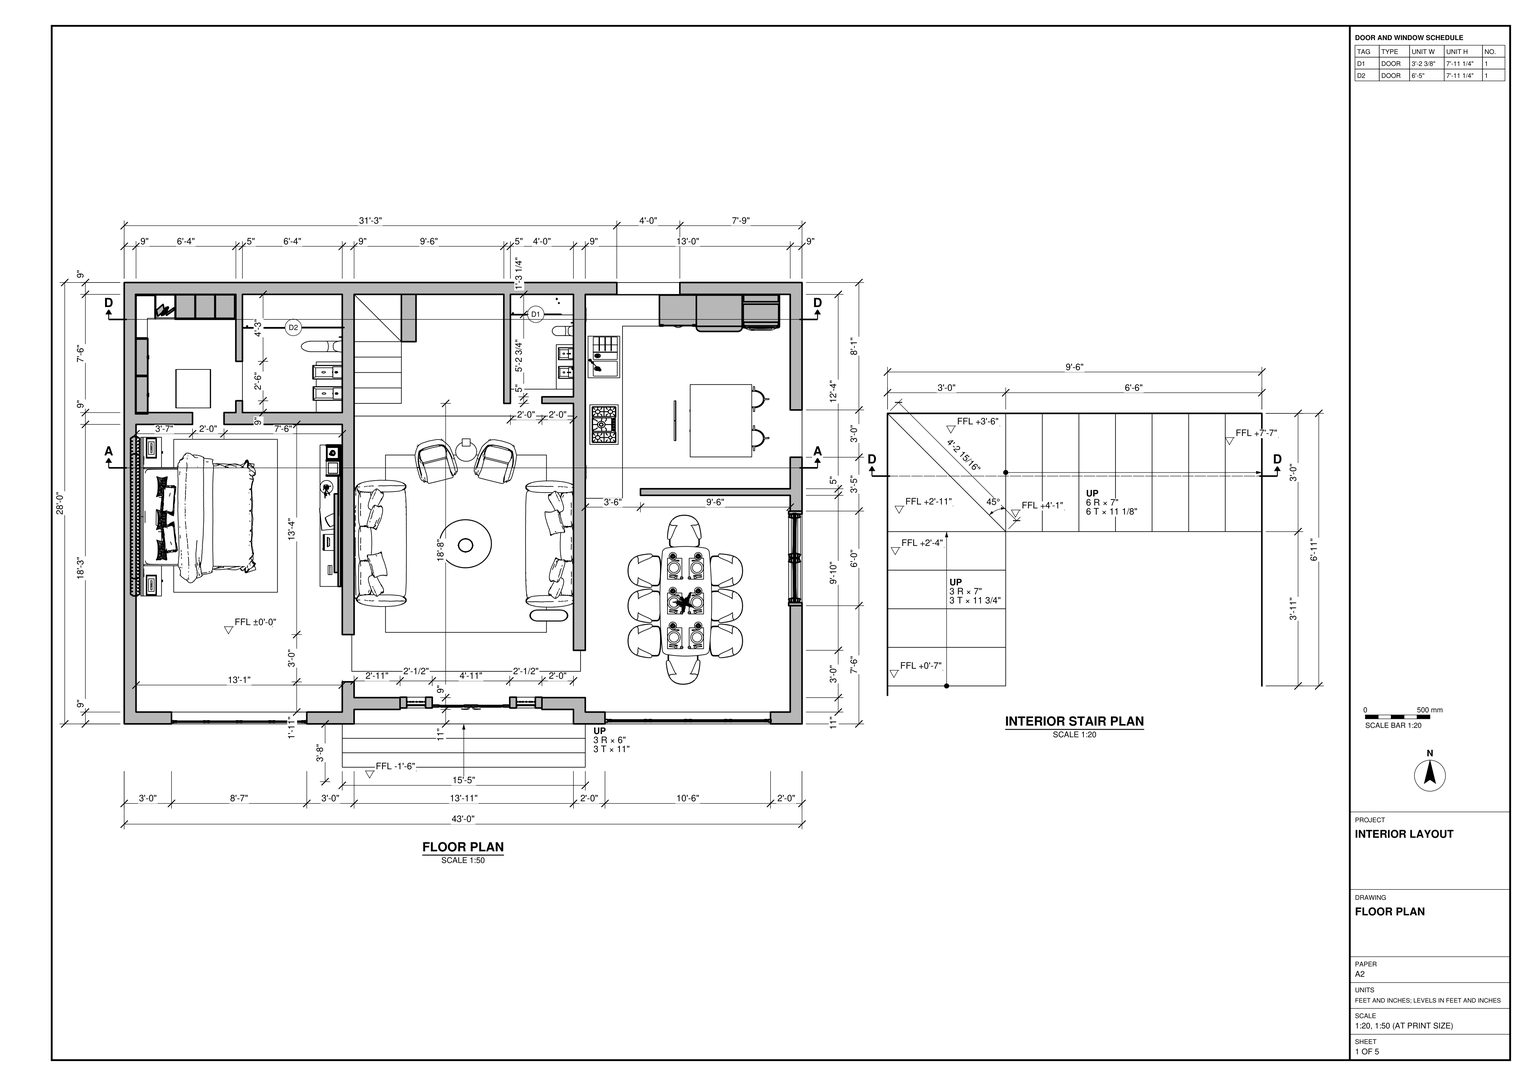
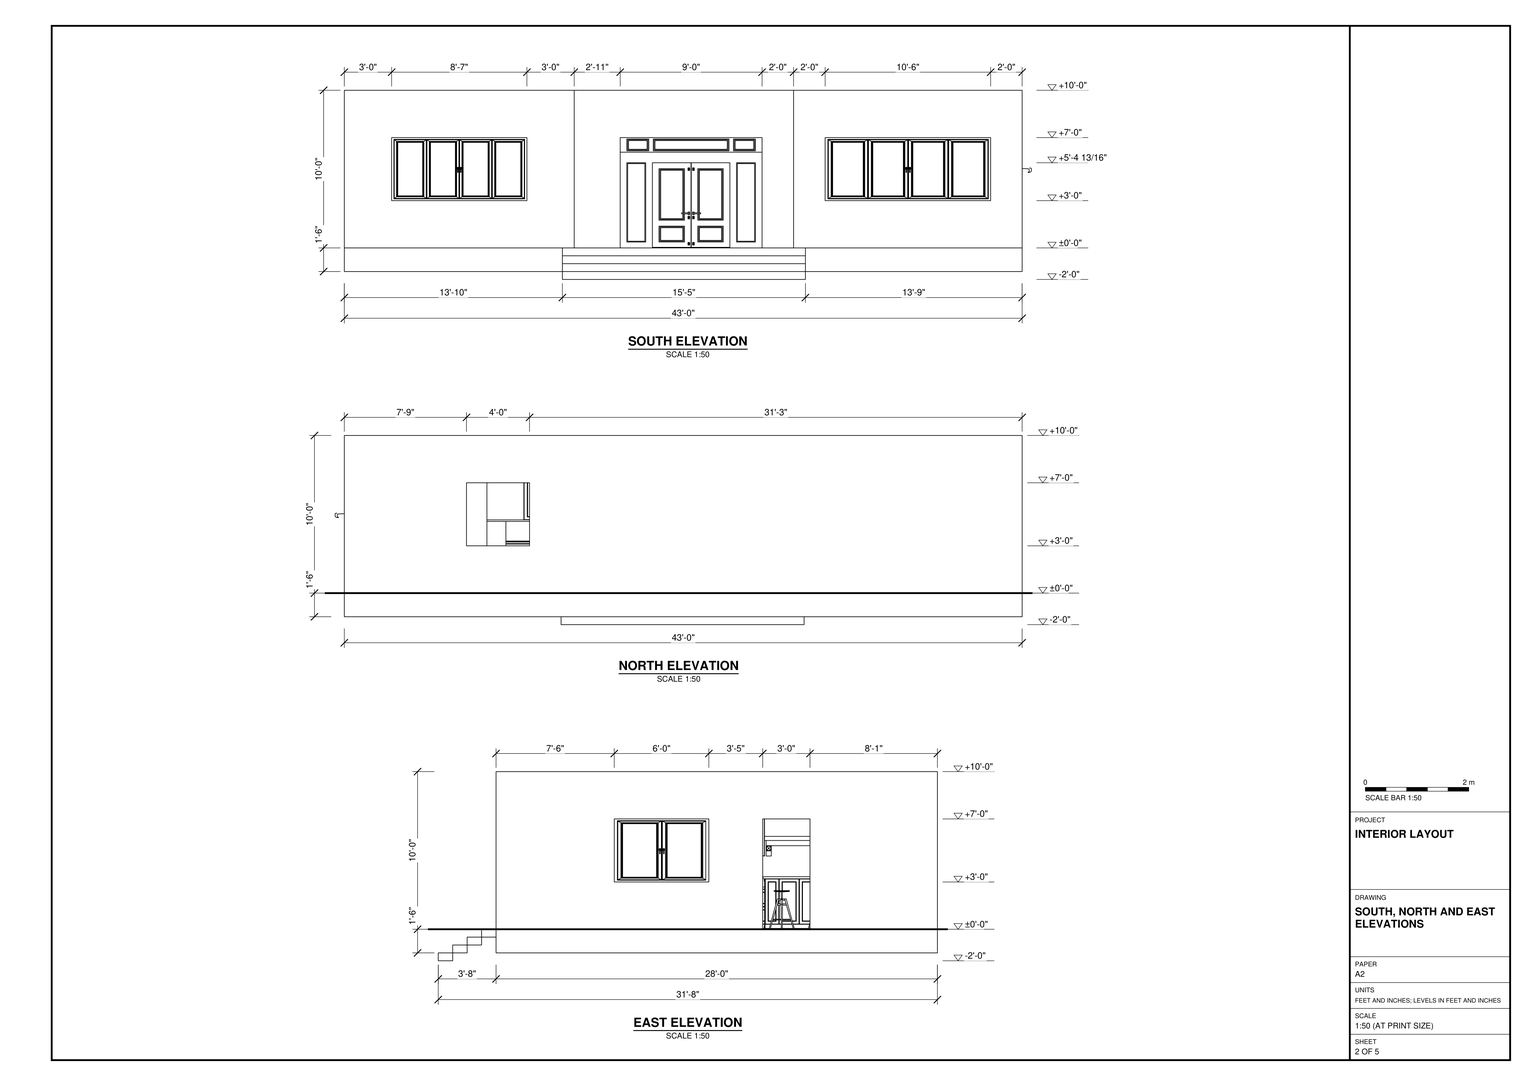
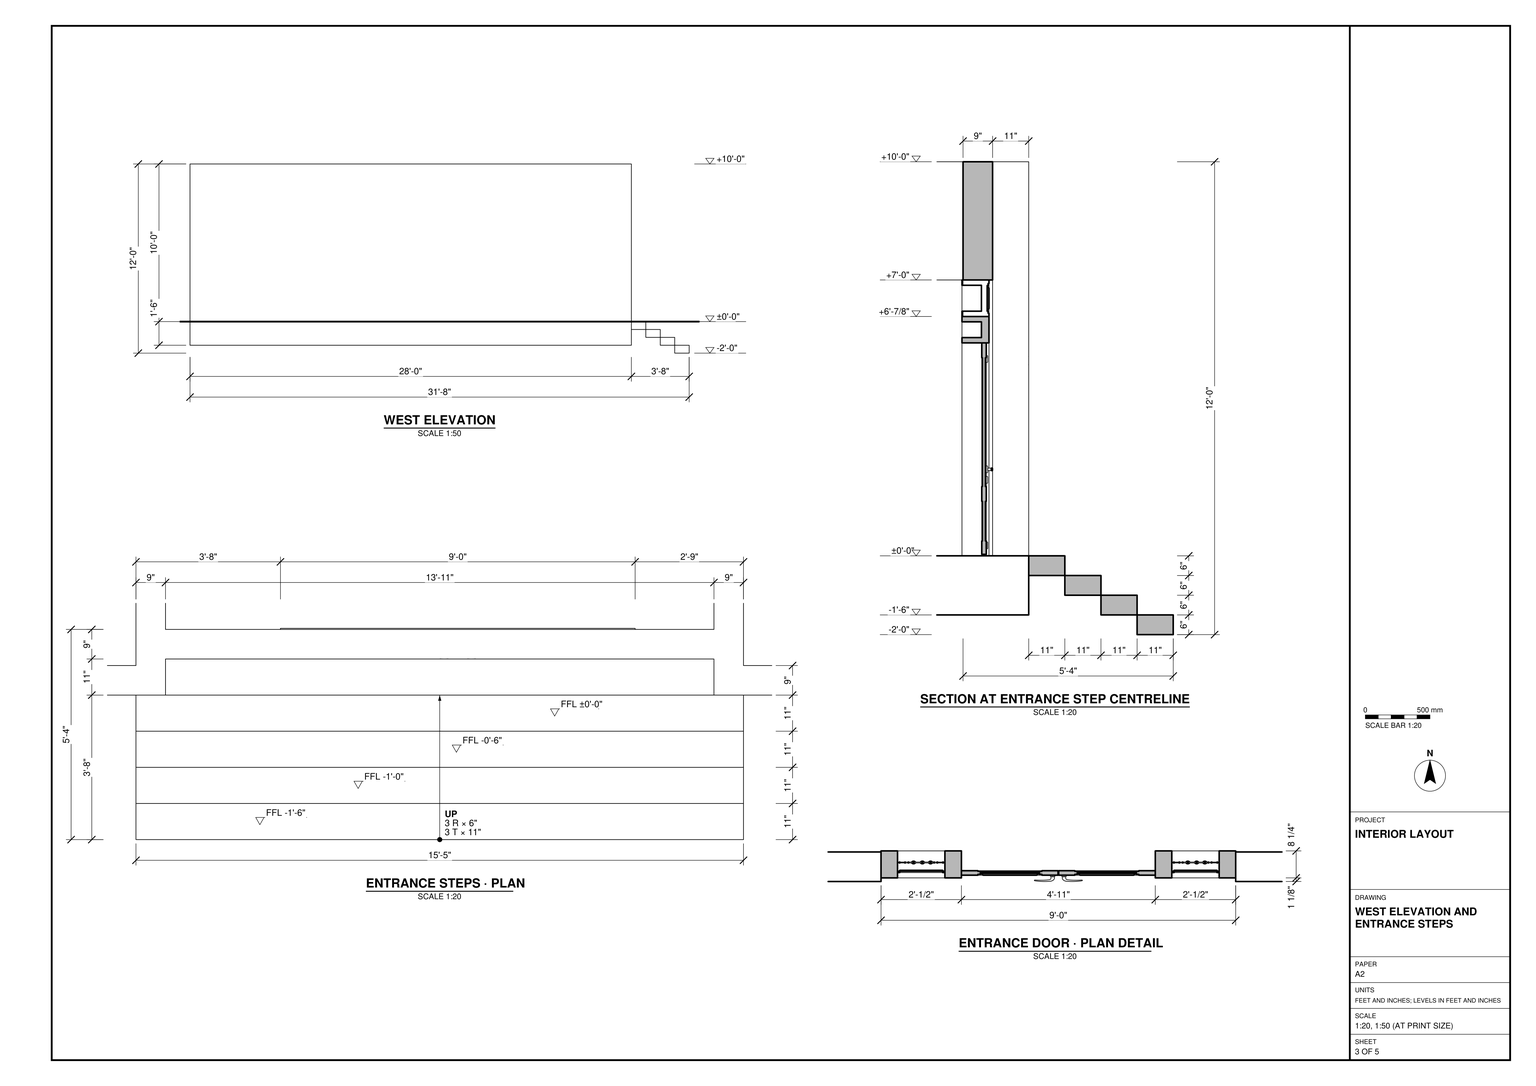
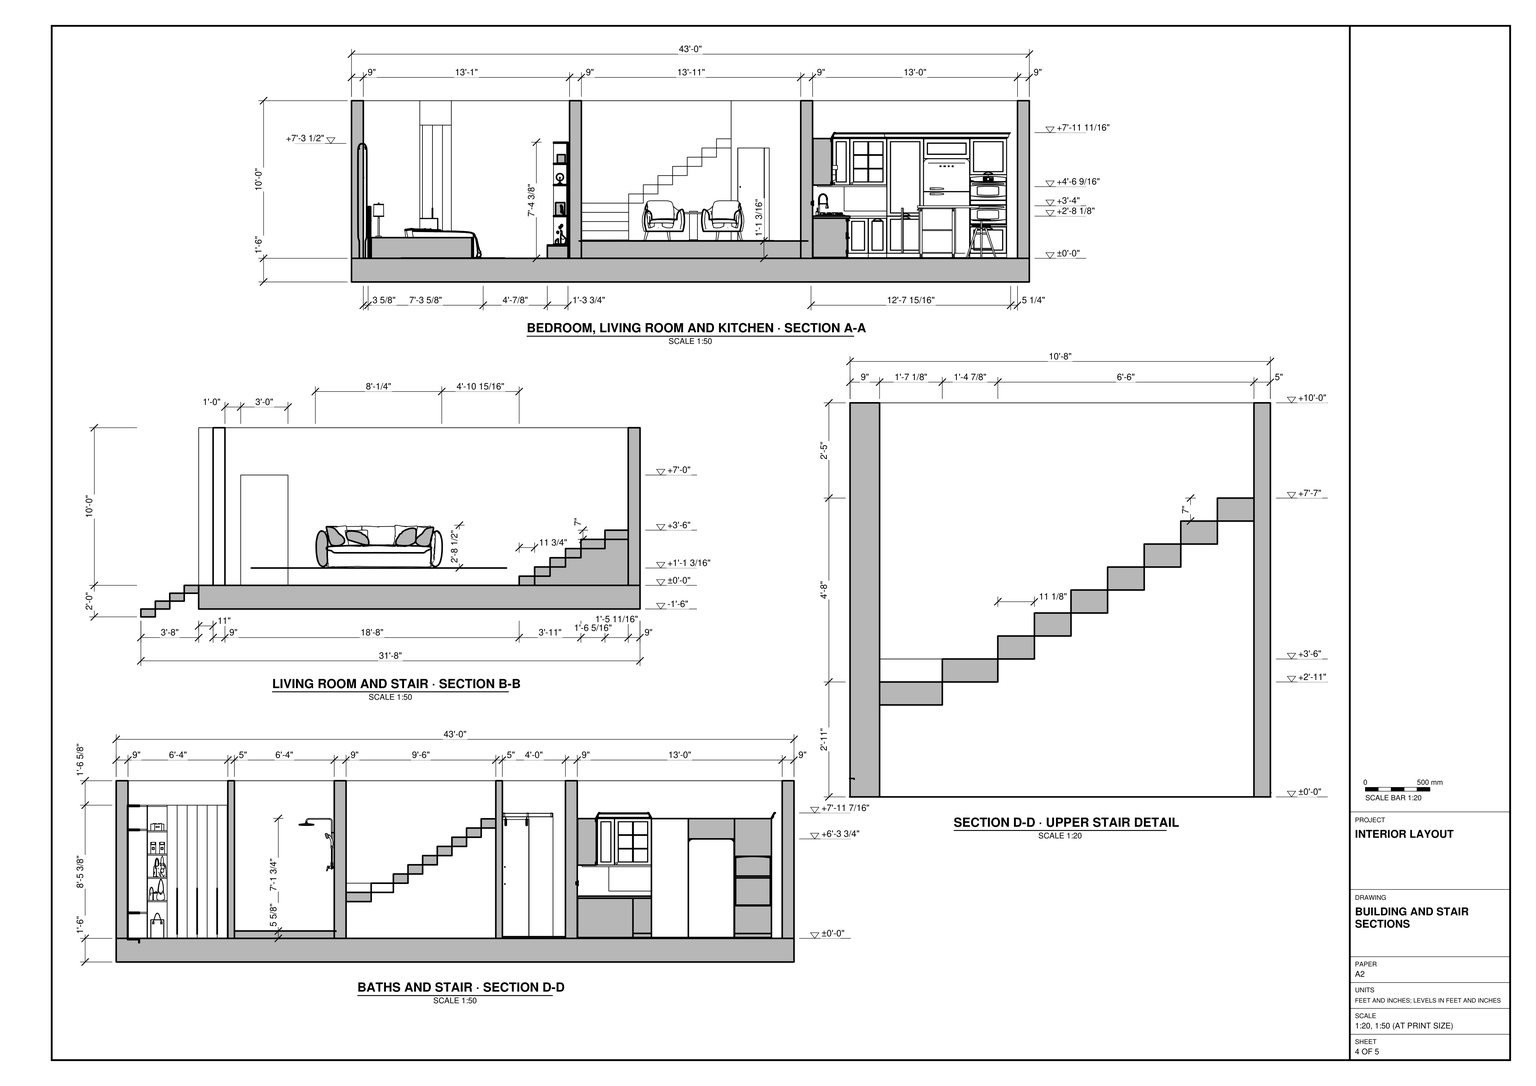
Build the residential interior in SketchUp from task_files/diagram_01.pdf. Work in feet and inches. The complete model measures 43'-7 7/16" along X, 40'-11 11/16" along Y and 12'-0" vertically. Set the finished ground floor at ±0'-0". Distinguish the complete model extents from the 43'-0" by 28'-0" exterior wall footprint on the floor plan.

Model the raised floor slab, the 9" exterior walls and the interior walls at their drawn thicknesses, including the 5" partitions. Form the recessed south entrance with broad steps, paired door leaves, sidelights and a transom. Use the elevations to locate the window units and the openings on the east and north walls. Model the interior stair behind the living area, including the angled treads where the flight turns.

Place the bed with its head against the west wall, bedside units on either side and storage opposite. Fit out the small rooms along the north wall with the storage and sanitary fixtures shown. Arrange the central sofas facing each other across the round table, with the armchairs toward the stair. In the east bay, model the kitchen counters, sink, cooktop, island and stools behind the dining area. Match the footprints and orientations of the dining table, chairs and other main furniture to the plan. Decor and loose items may be any suitable library components.

Keep the shell elements, stairs and each furniture or joinery piece in separate groups or components, and use components for repeated parts. Save one SketchUp model as output_files/furnished_interior_with_entrance_steps_and_turning_stair.skp.

# SketchUp Ruby script. Lengths in inches.
U = 1.inch
M = Sketchup.active_model
def pt(a) = Geom::Point3d.new(a.map { |v| v * U })
def face(e, loops, mat)
  f = e.add_face(loops[0].map { |a| pt(a) })
  loops[1..].each { |l| e.add_face(l.map { |a| pt(a) }).erase! }
  f.material = f.back_material = mat if mat
  f
end
# faces: each face lists its corners as indices into pts; further lists are holes
def faces(e, pts, list, mat = nil) = list.each { |f| face(e, (f[0].is_a?(Array) ? f : [f]).map { |l| l.map { |i| pts[i] } }, mat) }
# xy, xz, yz: faces in a plane at the given z, y or x. An outline is a flat list of corners, or four numbers for a rectangle; further outlines are holes
def ring(l) = l.size == 4 ? [[l[0], l[1]], [l[2], l[1]], [l[2], l[3]], [l[0], l[3]]] : l.each_slice(2).to_a
def flat(e, list, mat, &to3) = list.each { |f| face(e, (f[0].is_a?(Array) ? f : [f]).map { |l| ring(l).map { |u, v| to3.(u, v) } }, mat) }
def xy(e, z, list, mat = nil) = flat(e, list, mat) { |x, y| [x, y, z] }
def xz(e, y, list, mat = nil) = flat(e, list, mat) { |x, z| [x, y, z] }
def yz(e, x, list, mat = nil) = flat(e, list, mat) { |y, z| [x, y, z] }
def lines(e, pts, list) = list.each { |a, b| e.add_line(pt(pts[a]), pt(pts[b])) }
# prism: a flat outline (further loops are holes) pulled along v
def prism(e, loops, v, mat = nil)
  f = face(e, loops, mat); d = Geom::Vector3d.new(v.map { |x| x * U })
  f.pushpull(f.normal.samedirection?(d) ? d.length : -d.length)
end
def box(e, o, s, mat = nil) = prism(e, [[o, [o[0] + s[0], o[1], o[2]], [o[0] + s[0], o[1] + s[1], o[2]], [o[0], o[1] + s[1], o[2]]]], [0, 0, s[2]], mat)
def at(x, y, z, deg = 0) = Geom::Transformation.translation(pt([x, y, z])) * Geom::Transformation.rotation(ORIGIN, Z_AXIS, deg.degrees)
def axes(o, x, y, z) = Geom::Transformation.new([*x, 0, *y, 0, *z, 0, *pt(o).to_a, 1])
def part(name) = M.definitions.add(name)
# library, detail: a bought-in or finely detailed component or shape, given as its bounding box
def library(name, o, s) = part(name).tap { |d| box(d.entities, o, s) }
def detail(e, o, s) = box(e.add_group.entities, o, s)
def put(e, d, t, mat = nil) = e.add_instance(d, t).tap { |i| i.material = mat if mat }
def group(e, t, mat = nil) = e.add_group.tap { |g| g.transformation = t; g.material = mat if mat }.entities
root = M.entities
M.materials.add("02").color = [126, 126, 126]
M.materials.add("9225458-white-marble-texture-background-High-resolution-scan").color = [224, 224, 224]
M.materials.add("Hairline Grey").color = [62, 62, 62]
M.materials.add("Lisanne_Boots").color = [231, 232, 226]
M.materials.add("WD-03").color = [28, 27, 25]
M.materials.add("WoodPlanksClean0025_9_S").color = [124, 95, 68]
M.materials.add("[0100_SteelBlue]").color = [246, 244, 236]
M.materials.add("[0131_Silver]").color = [192, 192, 192]
M.materials.add("[Aluminum]").color = [179, 179, 179]
M.materials.add("[Blacktop Old 01]").color = [132, 136, 139]
M.materials.add("[Carrera Marble]").color = [207, 207, 207]
M.materials.add("[Granite Brown]").color = [126, 104, 91]
M.materials.add("[Roofing Slate Tan]").color = [200, 175, 128]
M.materials.add("[Slate Light Tile]").color = [54, 54, 54]
M.materials.add("[Stone Vein Gray]").color = [166, 165, 165]
M.materials.add("[Tile Large Brown]").color = [195, 178, 159]
M.materials.add("[Translucent Glass Gray]").color = [128, 128, 128]
M.materials["[Translucent Glass Gray]"].alpha = 0.5
M.materials.add("trees-164929_960_1").color = [98, 98, 98]
c1 = library("K-3091 Purist(R) Mirrored Cabinet",[0,-6.88,-2.03],[25.45,6.88,38.03])
c2 = library("Sink",[-425.26,-17.96,-2.45],[19.83,19.83,15.37])
c3 = library("CS761DT5",[0,0,0],[27.72,16.22,33.63])
c4 = library("SHOWER",[23.01,60.26,14.57],[13.03,23.97,40.35])
c5 = part("Bar")
prism(c5.entities,[[[0,0.25,0.5],[0,0.47,0.375],[0,0.47,0.125],[0,0.25,0],[0,0.03,0.125],[0,0.03,0.375]]],[11.5,0,0])
c6 = part("End")
xy(c6.entities,0,[[0,0.25,0.875,1.5]],"[0131_Silver]")
xy(c6.entities,0.5,[[0,0.25,0.875,1.5]],"[0131_Silver]")
xz(c6.entities,0.03,[[0,0.125,0.25,0.375]],"[0131_Silver]")
xz(c6.entities,0.47,[[0.25,0.125,0.875,0.375]],"[0131_Silver]")
xz(c6.entities,1.5,[[0,0,0.875,0.5]],"[0131_Silver]")
yz(c6.entities,0,[[0.25,0,0.03,0.125,0.03,0.375,0.25,0.5,1.5,0.5,1.5,0]],"[0131_Silver]")
yz(c6.entities,0.25,[[0.25,0,0.47,0.125,0.47,0.375,0.25,0.5,0.03,0.375,0.03,0.125]],"[0131_Silver]")
yz(c6.entities,0.875,[[0.25,0,1.5,0,1.5,0.5,0.25,0.5,0.47,0.375,0.47,0.125]],"[0131_Silver]")
p = [[0,0.25,0],[0.25,0.25,0],[0.25,0.03,0.125],[0,0.03,0.125],[0.875,0.25,0],[0.875,0.47,0.125],
  [0.25,0.47,0.125],[0,0.03,0.375],[0.25,0.03,0.375],[0.25,0.25,0.5],[0,0.25,0.5],[0.875,0.47,0.375],
  [0.875,0.25,0.5],[0.25,0.47,0.375]]
faces(c6.entities,p,[[0,1,2,3],[4,5,6,1],[7,8,9,10],[11,12,9,13]],"[0131_Silver]")
c7 = part("Drawer Pull\#2")
put(c7.entities,c5,axes([0.25,0,0],[1.16,0,0],[0,0.76843,0],[0,0,1]),"[0131_Silver]")
put(c7.entities,c6,axes([0,0,0],[1,0,0],[0,1.02284,0],[0,0,1]))
put(c7.entities,c6,axes([13.84,0,0],[-1,0,0],[0,1.02284,0],[0,0,1]))
c8 = part("NUT")
prism(c8.entities,[[[0.34,0,0],[0,0.2,0],[0,0.6,0],[0.34,0.79,0],[0.6875,0.6,0],[0.6875,0.2,0]]],[0,0,0.25])
c9 = part("BOLT HEAD")
yz(c9.entities,0,[[0.34,-0.14,0.27,-0.12,0.22,-0.07,0.21,0,0.22,0.07,0.27,0.12,0.34,0.14,0.41,0.12,0.46,0.07,0.48,0,0.46,-0.07,0.41,-0.12]])
p = [[0.1875,0.05,-0.17],[0,0.22,-0.07],[0,0.27,-0.12],[0.1875,0.17,-0.3],[0,0.34,-0.14],[0.1875,0.34,-0.34],
  [0,0.41,-0.12],[0.1875,0.52,-0.3],[0,0.46,-0.07],[0.1875,0.64,-0.17],[0.1875,0,0],[0,0.21,0],
  [0,0.48,0],[0.1875,0.6875,0],[0.1875,0.05,0.17],[0,0.22,0.07],[0,0.46,0.07],[0.1875,0.64,0.17],
  [0.1875,0.17,0.3],[0,0.27,0.12],[0.1875,0.34,0.34],[0,0.34,0.14],[0.1875,0.52,0.3],[0,0.41,0.12]]
faces(c9.entities,p,[[0,1,2,3],[3,2,4,5],[5,4,6,7],[7,6,8,9],[10,11,1,0],[9,8,12,13],[14,15,11,10],[13,12,16,17],
  [18,19,15,14],[20,21,19,18],[22,23,21,20],[17,16,23,22]])
c10 = part("Group\#42")
xy(c10.entities,0,[[0.33,0.41,0.33,0.75,0,0.97,0,1.4375,0.19,1.4375,0.19,1.07,0.52,0.85,0.52,0.41],[0,1.4375,0,1.91,0.33,2.12,0.33,2.46,0.52,2.46,0.52,2.02,0.19,1.8,0.19,1.4375]],"[Aluminum]")
xy(c10.entities,4.24,[[0.625,0,1.0625,0.85],[0.625,2.02,1.0625,2.875]],"[Aluminum]")
xy(c10.entities,4.43,[[0.6,0,1.0625,0.75],[0.6,2.12,1.0625,2.875]],"[Aluminum]")
xy(c10.entities,4.57,[[0.58,1.07,1.0625,1.4375],[0.58,1.4375,1.0625,1.8]],"[Aluminum]")
xy(c10.entities,4.76,[[0.56,0.97,1.0625,1.4375],[0.56,1.4375,1.0625,1.91]],"[Aluminum]")
xz(c10.entities,0,[[0.33,0.41,0.52,0.41,0.52,4.14,0.53,4.1875,0.57,4.23,0.625,4.24,1.0625,4.24,1.0625,4.43,0.6,4.43,0.47,4.4,0.36,4.29,0.33,4.16]],"[Aluminum]")
xz(c10.entities,2.875,[[0.33,0.41,0.33,4.16,0.36,4.29,0.47,4.4,0.6,4.43,1.0625,4.43,1.0625,4.24,0.625,4.24,0.57,4.23,0.53,4.1875,0.52,4.14,0.52,0.41]],"[Aluminum]")
yz(c10.entities,0,[[0.97,0,1.4375,4.2],[1.4375,0,1.91,4.2]],"[Aluminum]")
yz(c10.entities,0.19,[[1.07,0,1.4375,4.18],[1.4375,0,1.8,4.18]],"[Aluminum]")
yz(c10.entities,0.33,[[0.41,0,0,0.41,0,4.16,0.75,4.16,0.75,0],[2.12,0,2.12,4.16,2.875,4.16,2.875,0.41,2.46,0]],"[Aluminum]")
yz(c10.entities,0.52,[[0.41,0,0.85,0,0.85,4.14,0,4.14,0,0.41],[2.02,0,2.46,0,2.875,0.41,2.875,4.14,2.02,4.14]],"[Aluminum]")
yz(c10.entities,1.0625,[[0,4.24,0.85,4.24,1.07,4.57,1.4375,4.57,1.4375,4.76,0.97,4.76,0.75,4.43,0,4.43],[2.02,4.24,2.875,4.24,2.875,4.43,2.12,4.43,1.91,4.76,1.4375,4.76,1.4375,4.57,1.8,4.57]],"[Aluminum]")
p = [[0.33,0,0.41],[0.33,0.41,0],[0.52,0.41,0],[0.52,0,0.41],[0,0.97,0],[0.33,0.75,0],
  [0.33,0.75,4.16],[0,0.97,4.2],[0.52,0.85,0],[0.19,1.07,0],[0.19,1.07,4.18],[0.52,0.85,4.14],
  [0.19,1.8,0],[0.52,2.02,0],[0.52,2.02,4.14],[0.19,1.8,4.18],[0.33,2.12,0],[0,1.91,0],
  [0,1.91,4.2],[0.33,2.12,4.16],[0.33,2.46,0],[0.33,2.875,0.41],[0.52,2.875,0.41],[0.52,2.46,0],
  [0.52,0,4.14],[0.53,0.85,4.1875],[0.53,0,4.1875],[0.24,1.07,4.36],[0.53,2.02,4.1875],[0.24,1.8,4.36],
  [0.52,2.875,4.14],[0.53,2.875,4.1875],[0.33,0,4.16],[0.36,0,4.29],[0.36,0.75,4.29],[0.57,0.85,4.23],
  [0.57,0,4.23],[0.625,0.85,4.24],[0.625,0,4.24],[0.07,0.97,4.46],[0.4,1.07,4.52],[0.58,1.07,4.57],
  [1.0625,1.07,4.57],[1.0625,0.85,4.24],[0.07,1.4375,4.46],[0,1.4375,4.2],[0.19,1.4375,4.18],[0.24,1.4375,4.36],
  [0.07,1.91,4.46],[0.57,2.02,4.23],[0.4,1.8,4.52],[0.625,2.02,4.24],[0.58,1.8,4.57],[1.0625,2.02,4.24],
  [1.0625,1.8,4.57],[0.36,2.12,4.29],[0.57,2.875,4.23],[0.625,2.875,4.24],[0.33,2.875,4.16],[0.36,2.875,4.29],
  [0.47,0,4.4],[0.47,0.75,4.4],[0.3,0.97,4.69],[0.3,1.91,4.69],[0.47,2.12,4.4],[0.47,2.875,4.4],
  [0.6,0,4.43],[0.6,0.75,4.43],[0.56,0.97,4.76],[1.0625,0.75,4.43],[1.0625,0.97,4.76],[0.4,1.4375,4.52],
  [0.56,1.91,4.76],[0.6,2.12,4.43],[1.0625,1.91,4.76],[1.0625,2.12,4.43],[0.6,2.875,4.43],[0.3,1.4375,4.69],
  [0.58,1.4375,4.57],[0.56,1.4375,4.76]]
faces(c10.entities,p,[[0,1,2,3],[4,5,6,7],[8,9,10,11],[12,13,14,15],[16,17,18,19],[20,21,22,23],[24,11,25,26],[11,10,27,25],
  [15,14,28,29],[14,30,31,28],[6,32,33,34],[26,25,35,36],[36,35,37,38],[7,6,34,39],[25,27,40,35],[35,40,41,37],
  [37,41,42,43],[39,44,45,7],[10,46,47,27],[44,48,18,45],[46,15,29,47],[29,28,49,50],[50,49,51,52],[52,51,53,54],
  [19,18,48,55],[28,31,56,49],[49,56,57,51],[58,19,55,59],[34,33,60,61],[39,34,61,62],[55,48,63,64],[59,55,64,65],
  [61,60,66,67],[62,61,67,68],[68,67,69,70],[27,47,71,40],[47,29,50,71],[64,63,72,73],[73,72,74,75],[65,64,73,76],
  [62,77,44,39],[40,71,78,41],[77,63,48,44],[71,50,52,78],[68,79,77,62],[79,72,63,77]],"[Aluminum]")
put(c10.entities,c9,at(0.14,0.03,3),"[Aluminum]")
put(c10.entities,c9,axes([0.14,2.84,1],[1,0,0],[0,-1,0],[0,0,1]),"[Aluminum]")
put(c10.entities,c9,at(0.14,0.03,1),"[Aluminum]")
put(c10.entities,c9,axes([0.14,2.84,3],[1,0,0],[0,-1,0],[0,0,1]),"[Aluminum]")
c11 = part("Group\#43")
put(c11.entities,c10,at(0,0.01,0))
put(c11.entities,c10,axes([1.77,2.88,0],[-0.99999,-0.00487,0.00008],[0.00487,-0.99999,0],[0.00008,0,1]))
c12 = part("Shower Barn Door\#2")
put(c12.entities,c7,axes([29.5,51.24,54.55],[0,0,-1],[-1,0,0],[0,1,0]))
g1 = group(c12.entities,at(27.51,49.73,-0.07))
prism(g1,[[[0,18.67,92.1875],[0,18.67,95.27],[1.63,18.67,95.27],[1.63,18.67,92.1875],[1.01,18.67,92.1875],[1.01,18.67,92.3],[1.54,18.67,92.3],[1.54,18.67,95.125],[0.1,18.67,95.125],[0.1,18.67,92.3],[0.625,18.67,92.3],[0.625,18.67,92.1875]]],[0,1.06,0],"[Aluminum]")
prism(g1,[[[0.94,18.42,91.36],[0.96,18.37,91.36],[0.94,18.32,91.36],[0.89,18.28,91.36],[0.82,18.27,91.36],[0.74,18.28,91.36],[0.69,18.32,91.36],[0.67,18.37,91.36],[0.69,18.42,91.36],[0.74,18.45,91.36],[0.82,18.47,91.36],[0.89,18.45,91.36]]],[0,0,1.3],"[Aluminum]")
prism(g1,[[[0.94,2.45,91.36],[0.96,2.4,91.36],[0.94,2.35,91.36],[0.89,2.3125,91.36],[0.82,2.3,91.36],[0.74,2.3125,91.36],[0.69,2.35,91.36],[0.67,2.4,91.36],[0.69,2.45,91.36],[0.74,2.48,91.36],[0.82,2.5,91.36],[0.89,2.48,91.36]]],[0,0,1.31],"[Aluminum]")
xy(g1,0,[[0.86,19.93,0.96,38.4]])
xy(g1,0.07,[[0.64,0,0.73,20.16]])
xy(g1,92.15,[[0,0.57,0.625,1.64],[1.01,0.57,1.63,1.64]],"[Aluminum]")
xy(g1,92.1875,[[0,36.77,0.625,37.83],[1.01,36.77,1.63,37.83]],"[Aluminum]")
xy(g1,92.3,[[0.1,0.57,0.625,1.64],[1.01,0.57,1.54,1.64]],"[Aluminum]")
xy(g1,92.33,[[0.1,36.77,0.625,37.83],[1.01,36.77,1.54,37.83]],"[Aluminum]")
xy(g1,95.125,[[0.1,0.57,1.54,1.64],[0.1,36.77,1.54,37.83]],"[Aluminum]")
xy(g1,95.27,[[0,0.57,1.63,1.64],[0,36.77,1.63,37.83]],"[Aluminum]")
xz(g1,0,[[0.64,0.07,0.73,90.26]],"[Translucent Glass Gray]")
xz(g1,0.57,[[0,92.15,0,95.27,1.63,95.27,1.63,92.15,1.01,92.15,1.01,92.3,1.54,92.3,1.54,95.125,0.1,95.125,0.1,92.3,0.625,92.3,0.625,92.15]],"[Aluminum]")
xz(g1,1.64,[[0,92.15,0.625,92.15,0.625,92.3,0.1,92.3,0.1,95.125,1.54,95.125,1.54,92.3,1.01,92.3,1.01,92.15,1.63,92.15,1.63,95.27,0,95.27]])
xz(g1,19.93,[[0.86,0,0.96,92.58]],"[Translucent Glass Gray]")
xz(g1,20.16,[[0.64,0.07,0.73,90.29]],"[Translucent Glass Gray]")
xz(g1,36.77,[[0,92.1875,0,95.27,1.63,95.27,1.63,92.1875,1.01,92.1875,1.01,92.33,1.54,92.33,1.54,95.125,0.1,95.125,0.1,92.33,0.625,92.33,0.625,92.1875]])
xz(g1,37.83,[[0,92.1875,0.625,92.1875,0.625,92.33,0.1,92.33,0.1,95.125,1.54,95.125,1.54,92.33,1.01,92.33,1.01,92.1875,1.63,92.1875,1.63,95.27,0,95.27]],"[Aluminum]")
xz(g1,38.4,[[0.86,0,0.96,92.62]],"[Translucent Glass Gray]")
yz(g1,0,[[0.57,92.15,1.64,95.27],[36.77,92.1875,37.83,95.27]],"[Aluminum]")
yz(g1,0.1,[[0.57,92.3,1.64,95.125],[36.77,92.33,37.83,95.125]],"[Aluminum]")
yz(g1,0.625,[[0.57,92.15,1.64,92.3],[36.77,92.1875,37.83,92.33]],"[Aluminum]")
yz(g1,0.64,[[0,0.07,0,90.26,20.16,90.29,20.16,0.07]],"[Translucent Glass Gray]")
yz(g1,0.73,[[0,0.07,20.16,0.07,20.16,90.29,0,90.26]],"[Translucent Glass Gray]")
yz(g1,0.86,[[19.93,0,19.93,92.58,38.4,92.62,38.4,0]],"[Translucent Glass Gray]")
yz(g1,0.96,[[19.93,0,38.4,0,38.4,92.62,19.93,92.58]],"[Translucent Glass Gray]")
yz(g1,1.01,[[0.57,92.15,1.64,92.3],[36.77,92.1875,37.83,92.33]],"[Aluminum]")
yz(g1,1.54,[[0.57,92.3,1.64,95.125],[36.77,92.33,37.83,95.125]],"[Aluminum]")
yz(g1,1.63,[[0.57,92.15,1.64,95.27],[36.77,92.1875,37.83,95.27]],"[Aluminum]")
p = [[0.64,20.16,90.29],[0.64,0,90.26],[0.73,0,90.26],[0.73,20.16,90.29],[0.86,38.4,92.62],[0.86,19.93,92.58],
  [0.96,19.93,92.58],[0.96,38.4,92.62]]
faces(g1,p,[[0,1,2,3],[4,5,6,7]])
put(g1,c8,axes([0.51,18.55,91.07],[0,-0.5323,0],[0.76843,0,0],[0,0,1.16]),"[Aluminum]")
put(g1,c8,axes([0.51,2.58,91.07],[0,-0.5323,0],[0.76843,0,0],[0,0,1.16]),"[Aluminum]")
g2 = group(g1,at(1.54,0.04,92.3),"[Aluminum]")
prism(g2,[[[-0.53,0,0.36],[-0.53,0,0],[0,0,0],[0,0,2.75],[-1.44,0,2.75],[-1.44,0,0],[-0.91,0,0],[-0.91,0,0.36],[-1.06,0,0.36],[-1.06,0,0.14],[-1.34,0,0.14],[-1.34,0,2.61],[-0.1,0,2.61],[-0.1,0,0.14],[-0.38,0,0.14],[-0.38,0,0.36]]],[0,38.33,0])
put(g1,c11,axes([0.05,17.6,85.52],[0.76843,0,0],[0,0.5323,0],[0,0,1.16]))
put(g1,c11,axes([0.05,1.63,85.52],[0.76843,0,0],[0,0.5323,0],[0,0,1.16]))
c13 = library("Bidet, Shower spray, Grohe - Sena",[8.94,6.65,1.98],[2.22,3.26,25.53])
c14 = library("cage d_003\#1",[-500,-500,-0.07],[1000,1000,320.07])
c15 = library("CAGE ripia\#3",[-494,-494,300],[988,988,20])
c16 = part("skp1815")
put(c16.entities,c14,at(0,0,0))
put(c16.entities,c15,at(0,0,0))
c17 = part("WestElm_MosaicCircleRug")
g3 = group(c17.entities,at(8.54,10.125,0))
xy(g3,0,[[0,0,96,120]],"Lisanne_Boots")
xy(g3,0.125,[[0,0,96,120]])
xz(g3,0,[[0,0,96,0.125]],"Lisanne_Boots")
xz(g3,120,[[0,0,96,0.125]],"Lisanne_Boots")
yz(g3,0,[[0,0,120,0.125]],"Lisanne_Boots")
yz(g3,96,[[0,0,120,0.125]],"Lisanne_Boots")
c18 = library("Armchair",[-16.34,-19.23,-0.05],[32.68,37.4,30.76])
c19 = part("Cantilever side table")
g4 = group(c19.entities,at(12.79,20.67,0,180),"[0100_SteelBlue]")
xy(g4,22.64,[[0.59,0.2,7.28,6.89]])
xz(g4,0.2,[[0.59,0,7.28,22.64]])
xz(g4,6.89,[[0.59,0,7.28,22.64]])
yz(g4,0.59,[[0.2,0,6.89,22.64]])
yz(g4,7.28,[[0.2,0,6.89,22.64]])
g5 = group(c19.entities,at(16.73,16.73,20.75,180),"Hairline Grey")
xy(g5,0,[[[7.52,-0.98,6.97,-0.94,6.42,-0.87,5.87,-0.76,5.33,-0.62,4.81,-0.4375,4.29,-0.23,3.79,0.01,3.3,0.28,2.84,0.58,2.39,0.91,1.96,1.27,1.56,1.66,1.18,2.07,0.83,2.5,0.51,2.95,0.21,3.42,-0.05,3.91,-0.29,4.42,-0.49,4.9375,-0.65,5.47,-0.79,6.01,-0.89,6.55,-0.95,7.11,-0.98,7.66,-0.98,8.22,-0.94,8.77,-0.87,9.33,-0.76,9.87,-0.62,10.41,-0.4375,10.9375,-0.23,11.45,0.01,11.96,0.28,12.44,0.58,12.91,0.91,13.36,1.27,13.78,1.66,14.18,2.07,14.5625,2.5,14.91,2.95,15.24,3.42,15.53,3.91,15.8,4.42,16.03,4.9375,16.23,5.47,16.4,6.01,16.53,6.55,16.63,7.11,16.7,7.66,16.73,8.22,16.72,8.77,16.68,9.33,16.61,9.87,16.5,10.41,16.36,10.9375,16.18,11.45,15.97,11.96,15.73,12.44,15.46,12.91,15.16,13.36,14.83,13.78,14.47,14.18,14.09,14.5625,13.68,14.91,13.25,15.24,12.79,15.53,12.32,15.8,11.83,16.03,11.33,16.23,10.81,16.4,10.28,16.53,9.74,16.63,9.1875,16.7,8.64,16.73,8.08,16.72,7.52,16.68,6.97,16.61,6.42,16.5,5.87,16.36,5.33,16.18,4.81,15.97,4.29,15.73,3.79,15.46,3.3,15.16,2.84,14.83,2.39,14.47,1.96,14.09,1.56,13.68,1.18,13.25,0.83,12.79,0.51,12.32,0.21,11.83,-0.05,11.33,-0.29,10.81,-0.49,10.28,-0.65,9.74,-0.79,9.1875,-0.89,8.64,-0.95,8.08,-0.98],[7.5625,0,8.06,0,8.55,0.03,9.04,0.09,9.53,0.17,10.01,0.29,10.48,0.44,10.94,0.62,11.39,0.83,11.83,1.0625,12.25,1.32,12.65,1.61,13.03,1.92,13.4,2.26,13.74,2.62,14.06,3,14.35,3.39,14.62,3.8125,14.86,4.24,15.07,4.6875,15.26,5.15,15.42,5.62,15.54,6.09,15.64,6.58,15.7,7.07,15.74,7.5625,15.74,8.06,15.72,8.55,15.66,9.04,15.57,9.53,15.45,10.01,15.3,10.48,15.12,10.94,14.92,11.39,14.68,11.83,14.42,12.25,14.13,12.65,13.82,13.03,13.48,13.4,13.125,13.74,12.75,14.06,12.35,14.35,11.93,14.62,11.5,14.86,11.06,15.07,10.6,15.26,10.13,15.42,9.65,15.54,9.16,15.64,8.67,15.7,8.18,15.74,7.6875,15.74,7.19,15.72,6.7,15.66,6.21,15.57,5.73,15.45,5.26,15.3,4.8,15.12,4.35,14.92,3.92,14.68,3.5,14.42,3.09,14.13,2.71,13.82,2.35,13.48,2.01,13.125,1.6875,12.75,1.39,12.35,1.125,11.93,0.88,11.5,0.67,11.06,0.48,10.6,0.33,10.13,0.2,9.65,0.1,9.16,0.04,8.67,0,8.18,0,7.6875,0.03,7.19,0.09,6.7,0.17,6.21,0.29,5.73,0.44,5.26,0.62,4.8,0.83,4.35,1.0625,3.92,1.32,3.5,1.61,3.09,1.92,2.71,2.26,2.35,2.62,2.01,3,1.6875,3.39,1.39,3.8125,1.125,4.24,0.88,4.6875,0.67,5.15,0.48,5.62,0.33,6.09,0.2,6.58,0.1,7.07,0.04]],[7.5625,0,7.07,0.04,6.58,0.1,6.09,0.2,5.62,0.33,5.15,0.48,4.6875,0.67,4.24,0.88,3.8125,1.125,3.39,1.39,3,1.6875,2.62,2.01,2.26,2.35,1.92,2.71,1.61,3.09,1.32,3.5,1.0625,3.92,0.83,4.35,0.62,4.8,0.44,5.26,0.29,5.73,0.17,6.21,0.09,6.7,0.03,7.19,0,7.6875,0,8.18,0.04,8.67,0.1,9.16,0.2,9.65,0.33,10.13,0.48,10.6,0.67,11.06,0.88,11.5,1.125,11.93,1.39,12.35,1.6875,12.75,2.01,13.125,2.35,13.48,2.71,13.82,3.09,14.13,3.5,14.42,3.92,14.68,4.35,14.92,4.8,15.12,5.26,15.3,5.73,15.45,6.21,15.57,6.7,15.66,7.19,15.72,7.6875,15.74,8.18,15.74,8.67,15.7,9.16,15.64,9.65,15.54,10.13,15.42,10.6,15.26,11.06,15.07,11.5,14.86,11.93,14.62,12.35,14.35,12.75,14.06,13.125,13.74,13.48,13.4,13.82,13.03,14.13,12.65,14.42,12.25,14.68,11.83,14.92,11.39,15.12,10.94,15.3,10.48,15.45,10.01,15.57,9.53,15.66,9.04,15.72,8.55,15.74,8.06,15.74,7.5625,15.7,7.07,15.64,6.58,15.54,6.09,15.42,5.62,15.26,5.15,15.07,4.6875,14.86,4.24,14.62,3.8125,14.35,3.39,14.06,3,13.74,2.62,13.4,2.26,13.03,1.92,12.65,1.61,12.25,1.32,11.83,1.0625,11.39,0.83,10.94,0.62,10.48,0.44,10.01,0.29,9.53,0.17,9.04,0.09,8.55,0.03,8.06,0]])
xy(g5,0.98,[[7.52,-0.98,8.08,-0.98,8.64,-0.95,9.1875,-0.89,9.74,-0.79,10.28,-0.65,10.81,-0.49,11.33,-0.29,11.83,-0.05,12.32,0.21,12.79,0.51,13.25,0.83,13.68,1.18,14.09,1.56,14.47,1.96,14.83,2.39,15.16,2.84,15.46,3.3,15.73,3.79,15.97,4.29,16.18,4.81,16.36,5.33,16.5,5.87,16.61,6.42,16.68,6.97,16.72,7.52,16.73,8.08,16.7,8.64,16.63,9.1875,16.53,9.74,16.4,10.28,16.23,10.81,16.03,11.33,15.8,11.83,15.53,12.32,15.24,12.79,14.91,13.25,14.5625,13.68,14.18,14.09,13.78,14.47,13.36,14.83,12.91,15.16,12.44,15.46,11.96,15.73,11.45,15.97,10.9375,16.18,10.41,16.36,9.87,16.5,9.33,16.61,8.77,16.68,8.22,16.72,7.66,16.73,7.11,16.7,6.55,16.63,6.01,16.53,5.47,16.4,4.9375,16.23,4.42,16.03,3.91,15.8,3.42,15.53,2.95,15.24,2.5,14.91,2.07,14.5625,1.66,14.18,1.27,13.78,0.91,13.36,0.58,12.91,0.28,12.44,0.01,11.96,-0.23,11.45,-0.4375,10.9375,-0.62,10.41,-0.76,9.87,-0.87,9.33,-0.94,8.77,-0.98,8.22,-0.98,7.66,-0.95,7.11,-0.89,6.55,-0.79,6.01,-0.65,5.47,-0.49,4.9375,-0.29,4.42,-0.05,3.91,0.21,3.42,0.51,2.95,0.83,2.5,1.18,2.07,1.56,1.66,1.96,1.27,2.39,0.91,2.84,0.58,3.3,0.28,3.79,0.01,4.29,-0.23,4.81,-0.4375,5.33,-0.62,5.87,-0.76,6.42,-0.87,6.97,-0.94]],"WD-03")
xz(g5,-0.98,[[7.52,0,8.08,0.98]])
yz(g5,-0.98,[[7.66,0,8.22,0.98]])
p = [[7.52,-0.98,0.98],[6.97,-0.94,0.98],[6.97,-0.94,0],[7.52,-0.98,0],[8.64,-0.95,0.98],[8.08,-0.98,0.98],
  [8.08,-0.98,0],[8.64,-0.95,0],[9.1875,-0.89,0.98],[9.1875,-0.89,0],[6.42,-0.87,0.98],[5.87,-0.76,0.98],
  [5.87,-0.76,0],[6.42,-0.87,0],[9.74,-0.79,0.98],[9.74,-0.79,0],[5.33,-0.62,0.98],[5.33,-0.62,0],
  [10.28,-0.65,0.98],[10.28,-0.65,0],[10.81,-0.49,0.98],[10.81,-0.49,0],[4.81,-0.4375,0.98],[4.81,-0.4375,0],
  [11.33,-0.29,0.98],[11.33,-0.29,0],[4.29,-0.23,0.98],[4.29,-0.23,0],[11.83,-0.05,0.98],[11.83,-0.05,0],
  [3.79,0.01,0.98],[3.79,0.01,0],[12.32,0.21,0.98],[12.32,0.21,0],[3.3,0.28,0.98],[3.3,0.28,0],
  [12.79,0.51,0.98],[12.79,0.51,0],[2.84,0.58,0.98],[2.84,0.58,0],[13.25,0.83,0.98],[13.25,0.83,0],
  [2.39,0.91,0.98],[2.39,0.91,0],[13.68,1.18,0.98],[13.68,1.18,0],[1.96,1.27,0.98],[1.96,1.27,0],
  [14.09,1.56,0.98],[14.09,1.56,0],[1.56,1.66,0.98],[1.56,1.66,0],[14.47,1.96,0.98],[14.47,1.96,0],
  [1.18,2.07,0.98],[1.18,2.07,0],[14.83,2.39,0.98],[14.83,2.39,0],[0.83,2.5,0.98],[0.83,2.5,0],
  [15.16,2.84,0.98],[15.16,2.84,0],[0.51,2.95,0.98],[0.51,2.95,0],[15.46,3.3,0.98],[15.46,3.3,0],
  [0.21,3.42,0.98],[0.21,3.42,0],[15.73,3.79,0.98],[15.73,3.79,0],[-0.05,3.91,0.98],[-0.05,3.91,0],
  [15.97,4.29,0.98],[15.97,4.29,0],[-0.29,4.42,0.98],[-0.29,4.42,0],[16.18,4.81,0.98],[16.18,4.81,0],
  [-0.49,4.9375,0.98],[-0.49,4.9375,0],[16.36,5.33,0.98],[16.36,5.33,0],[-0.65,5.47,0.98],[-0.65,5.47,0],
  [16.5,5.87,0.98],[16.5,5.87,0],[-0.79,6.01,0.98],[-0.79,6.01,0],[16.61,6.42,0.98],[16.61,6.42,0],
  [-0.89,6.55,0.98],[-0.89,6.55,0],[16.68,6.97,0.98],[16.68,6.97,0],[-0.95,7.11,0.98],[-0.95,7.11,0],
  [16.72,7.52,0.98],[16.72,7.52,0],[-0.98,7.66,0.98],[-0.98,7.66,0],[16.73,8.08,0.98],[16.73,8.08,0],
  [16.7,8.64,0.98],[16.7,8.64,0],[-0.98,8.22,0.98],[-0.94,8.77,0.98],[-0.94,8.77,0],[-0.98,8.22,0],
  [16.63,9.1875,0.98],[16.63,9.1875,0],[-0.87,9.33,0.98],[-0.87,9.33,0],[16.53,9.74,0.98],[16.53,9.74,0],
  [-0.76,9.87,0.98],[-0.76,9.87,0],[16.4,10.28,0.98],[16.4,10.28,0],[-0.62,10.41,0.98],[-0.62,10.41,0],
  [16.23,10.81,0.98],[16.23,10.81,0],[-0.4375,10.9375,0.98],[-0.4375,10.9375,0],[16.03,11.33,0.98],[16.03,11.33,0],
  [-0.23,11.45,0.98],[-0.23,11.45,0],[15.8,11.83,0.98],[15.8,11.83,0],[0.01,11.96,0.98],[0.01,11.96,0],
  [15.53,12.32,0.98],[15.53,12.32,0],[0.28,12.44,0.98],[0.28,12.44,0],[15.24,12.79,0.98],[15.24,12.79,0],
  [0.58,12.91,0.98],[0.58,12.91,0],[14.91,13.25,0.98],[14.91,13.25,0],[0.91,13.36,0.98],[0.91,13.36,0],
  [14.5625,13.68,0.98],[14.5625,13.68,0],[1.27,13.78,0.98],[1.27,13.78,0],[14.18,14.09,0.98],[14.18,14.09,0],
  [1.66,14.18,0.98],[1.66,14.18,0],[13.78,14.47,0.98],[13.78,14.47,0],[2.07,14.5625,0.98],[2.07,14.5625,0],
  [13.36,14.83,0.98],[13.36,14.83,0],[2.5,14.91,0.98],[2.5,14.91,0],[12.91,15.16,0.98],[12.91,15.16,0],
  [2.95,15.24,0.98],[2.95,15.24,0],[3.42,15.53,0.98],[3.42,15.53,0],[12.44,15.46,0.98],[12.44,15.46,0],
  [3.91,15.8,0.98],[3.91,15.8,0],[11.96,15.73,0.98],[11.96,15.73,0],[11.45,15.97,0.98],[11.45,15.97,0],
  [4.42,16.03,0.98],[4.42,16.03,0],[4.9375,16.23,0.98],[4.9375,16.23,0],[10.9375,16.18,0.98],[10.9375,16.18,0],
  [5.47,16.4,0.98],[5.47,16.4,0],[10.41,16.36,0.98],[10.41,16.36,0],[6.01,16.53,0.98],[6.01,16.53,0],
  [9.87,16.5,0.98],[9.87,16.5,0],[6.55,16.63,0.98],[6.55,16.63,0],[9.33,16.61,0.98],[9.33,16.61,0],
  [7.11,16.7,0.98],[7.11,16.7,0],[8.77,16.68,0.98],[8.77,16.68,0],[7.66,16.73,0.98],[7.66,16.73,0],
  [8.22,16.72,0.98],[8.22,16.72,0]]
faces(g5,p,[[0,1,2,3],[4,5,6,7],[8,4,7,9],[10,11,12,13],[1,10,13,2],[14,8,9,15],[11,16,17,12],[18,14,15,19],
  [20,18,19,21],[16,22,23,17],[24,20,21,25],[22,26,27,23],[28,24,25,29],[26,30,31,27],[32,28,29,33],[30,34,35,31],
  [36,32,33,37],[34,38,39,35],[40,36,37,41],[38,42,43,39],[44,40,41,45],[42,46,47,43],[48,44,45,49],[46,50,51,47],
  [52,48,49,53],[50,54,55,51],[56,52,53,57],[54,58,59,55],[60,56,57,61],[58,62,63,59],[64,60,61,65],[62,66,67,63],
  [68,64,65,69],[66,70,71,67],[72,68,69,73],[70,74,75,71],[76,72,73,77],[74,78,79,75],[80,76,77,81],[78,82,83,79],
  [84,80,81,85],[82,86,87,83],[88,84,85,89],[86,90,91,87],[92,88,89,93],[90,94,95,91],[96,92,93,97],[94,98,99,95],
  [100,96,97,101],[102,100,101,103],[104,105,106,107],[108,102,103,109],[105,110,111,106],[112,108,109,113],[110,114,115,111],[116,112,113,117],
  [114,118,119,115],[120,116,117,121],[118,122,123,119],[124,120,121,125],[122,126,127,123],[128,124,125,129],[126,130,131,127],[132,128,129,133],
  [130,134,135,131],[136,132,133,137],[134,138,139,135],[140,136,137,141],[138,142,143,139],[144,140,141,145],[142,146,147,143],[148,144,145,149],
  [146,150,151,147],[152,148,149,153],[150,154,155,151],[156,152,153,157],[154,158,159,155],[160,156,157,161],[158,162,163,159],[162,164,165,163],
  [166,160,161,167],[164,168,169,165],[170,166,167,171],[172,170,171,173],[168,174,175,169],[174,176,177,175],[178,172,173,179],[176,180,181,177],
  [182,178,179,183],[180,184,185,181],[186,182,183,187],[184,188,189,185],[190,186,187,191],[188,192,193,189],[194,190,191,195],[192,196,197,193],
  [196,198,199,197],[198,194,195,199]])
g6 = group(c19.entities,at(12.79,16.73,0,180),"Hairline Grey")
box(g6,[0.39,0,0],[7.09,11.02,0.98])
c20 = library("Dining Table",[-4.14,-4.14,0],[95.74,137.21,49.0625])
c21 = library("11",[-1.41,0,-0.63],[151.96,155.26,95.68])
c22 = library("Кровать",[-17.4,-26.33,0],[117.11,127.46,87.48])
c23 = library("tv unit model",[-7.7,0,0],[29.4,107.72,88.39])
c24 = library("Multi-panel window",[0,0,0],[118.11,4.67,70.87])
c25 = library("Paired window",[0,0,0],[60.51,4.67,70.87])
c26 = library("Bugatti",[-16.45,-211.33,0.73],[86.12,180.03,60.69])
c27 = part("Group\#2")
box(c27.entities,[0,0,0],[185,11,6])
c28 = part("Group\#5")
box(c28.entities,[0,0,0],[36,11.75,7])
c29 = part("Group\#8")
box(c29.entities,[0,0,0],[11.14,36,7])
c30 = library("Group\#59",[0,0,0],[77.28,90,95.46])
c31 = library("Agrupar\#10",[0,0,1.97],[12.91,12.91,5])
c32 = library("Group5\#2",[-94.38,-174.86,-59.07],[122.21,105.99,32.47])
c33 = library("Group5\#1",[-94.38,-174.86,-59.07],[122.21,105.99,32.47])
c34 = part("Group\#86")
xy(c34.entities,0,[[[0,0,24.26,27.29],[0.79,0.79,23.47,26.51]]],"trees-164929_960_1")
xy(c34.entities,1.18,[[[0,0,24.26,27.29],[0.79,0.79,23.47,26.51]]],"trees-164929_960_1")
xz(c34.entities,0,[[0,0,24.26,1.18]],"trees-164929_960_1")
xz(c34.entities,0.79,[[0.79,0,23.47,0.39],[0.79,0.39,23.47,1.18]],"trees-164929_960_1")
xz(c34.entities,26.51,[[0.79,0,23.47,0.39],[0.79,0.39,23.47,1.18]],"trees-164929_960_1")
xz(c34.entities,27.29,[[0,0,24.26,1.18]],"trees-164929_960_1")
yz(c34.entities,0,[[0,0,27.29,1.18]],"trees-164929_960_1")
yz(c34.entities,0.79,[[0.79,0,26.51,0.39],[0.79,0.39,26.51,1.18]],"trees-164929_960_1")
yz(c34.entities,23.47,[[0.79,0,26.51,0.39],[0.79,0.39,26.51,1.18]],"trees-164929_960_1")
yz(c34.entities,24.26,[[0,0,27.29,1.18]],"trees-164929_960_1")
c35 = library("Group\#89",[0,0,0],[21.46,10.33,21.85])
c36 = library("Group\#373",[0,0,0],[185.04,110.04,105.91])
c37 = library("Group\#485",[0,0.18,0],[126.77,13.39,109.66])
xy(root,0.25,[[294,355.37,342,378]],"[Slate Light Tile]")
xy(root,1.25,[[294,298.8,294,355.37,342,355.37,342,298.8,318.73,298.8,318.73,298.83,296.91,298.83,296.91,298.8]],"[Tile Large Brown]")
xy(root,28.25,[[328.91,298.8,342,332.74]],"[Tile Large Brown]")
xy(root,31.25,[[328.91,298.8,342,332.74]],"[Blacktop Old 01]")
xz(root,332.74,[[328.91,28.25,342,31.25]],"[Blacktop Old 01]")
xz(root,355.37,[[294,0.25,342,1.25]],"[Slate Light Tile]")
xz(root,378,[[294,0,342,0.25]])
yz(root,328.91,[[298.8,28.25,332.74,31.25]],"[Blacktop Old 01]")
yz(root,342,[[355.37,0,378,0.25]])
p = [[206.68,150.28,13.36],[206.68,227.3125,13.36]]
lines(root,p,[[0,1]])
put(root,c1,axes([342,330.9,47.58],[0,-0.96487,0],[0.19253,0,0],[0,0,0.97]))
put(root,c2,axes([341.03,115.77,34.08],[0,-0.47143,0],[0.58379,0,0],[0,0,1]))
put(root,c2,axes([340.91,130.02,33.76],[0,-0.47143,0],[0.58379,0,0],[0,0,1]))
put(root,c3,axes([342,346.93,0.25],[-0.58379,0,0],[0,-0.47143,0],[0,0,1]))
put(root,c4,axes([283.73,380.99,28.84],[-0.01528,-0.46975,0.08017],[0.58359,-0.0123,0.0021],[0,0.03781,0.99678]))
put(root,c12,axes([244.4,327.36,0.26],[0,1,0],[1,0,0],[0,0,1]))
put(root,c13,axes([336.24,354.11,-0.25],[0,-0.47143,0],[0.58379,0,0],[0,0,1]))
put(root,c16,axes([259.77,181.14,13.21],[-0.03976,0,0],[0,-0.0368,0],[0,0,0.03663]),"9225458-white-marble-texture-background-High-resolution-scan")
put(root,c17,axes([332.36,260.08,13.19],[-1.27652,0,0],[0,-1.1252,0],[0,0,1.344]),"WoodPlanksClean0025_9_S")
put(root,c18,axes([236.52,244.75,13.11],[0.87374,0.21668,0],[-0.23412,0.80867,0],[0,0,1]))
put(root,c18,axes([283.49,244.6,13.11],[0.87374,-0.21668,0],[0.23412,0.80867,0],[0,0,1]))
put(root,c19,axes([252.3125,243.91,13.19],[0.90456,0,0],[0,0.8372,0],[0,0,1]))
put(root,c20,at(383.4,74.06,0))
put(root,c21,at(351.22,215.74,0.63))
put(root,c22,at(16.96,164.39,0))
put(root,c23,at(148.62,148.62,0))
put(root,c24,axes([366,44,36],[1.07,0,0],[0,1,0],[0,0,0.67733]))
put(root,c25,axes([522.98,206,36],[0,-1.18993,0],[-5.16687,0,0],[0,0,0.67733]))
put(root,c24,axes([36,44,36],[0.87207,0,0],[0,0.71071,0],[0,0,0.67733]))
put(root,c26,at(147.49,-95.21,-18,90))
put(root,c27,at(166,33,-6),"[Granite Brown]")
put(root,c27,at(166,22,-12),"[Granite Brown]")
put(root,c27,at(166,11,-18),"[Granite Brown]")
put(root,c27,at(166,0,-24),"[Granite Brown]")
g7 = group(root,at(0,44,-18))
xy(g7,0,[[0,0,516,336]])
xy(g7,18,[[0,0,516,336]],"[Roofing Slate Tan]")
xz(g7,0,[[0,0,516,18]])
xz(g7,336,[[0,0,516,18]])
yz(g7,0,[[0,0,336,18]])
yz(g7,516,[[0,0,336,18]])
g8 = group(root,at(175,288,0))
p = [[0,83,0],[36,47,0],[47.14,47,0],[47.14,83,0],[58.29,47,0],[69.43,47,0],
  [69.43,83,0],[80.57,47,0],[80.57,83,0],[91.71,47,0],[91.71,83,0],[102.86,47,0],
  [0,47,0],[58.29,83,0],[102.86,83,0],[0,11.75,0],[36,11.75,0],[114,47,0],
  [0,23.5,0],[36,23.5,0],[36,35.25,0],[0,35.25,0],[114,83,0],[0,0,0],
  [36,0,0],[36,83,0]]
lines(g8,p,[[0,1],[2,3],[2,4],[4,5],[5,6],[7,8],[7,9],[9,10],[9,11],[12,1],[4,13],[5,7],
  [11,14],[15,16],[11,17],[18,19],[19,20],[21,20],[17,22],[16,19],[20,1],[23,24],[24,16],[1,2],
  [1,25]])
put(root,c28,at(175,288,0),"[Stone Vein Gray]")
put(root,c28,at(175,299.75,7),"[Stone Vein Gray]")
put(root,c28,at(175,311.5,14),"[Stone Vein Gray]")
put(root,c28,at(175,323.25,21),"[Stone Vein Gray]")
g9 = group(root,at(175,335,28),"[Carrera Marble]")
prism(g9,[[[36,0,0],[0,0,0],[0,36,0]]],[0,0,7])
g10 = group(root,at(175,335,35),"[Carrera Marble]")
prism(g10,[[[0,36,0],[36,36,0],[36,0,0]]],[0,0,7])
put(root,c29,at(211,335,42),"[Stone Vein Gray]")
put(root,c29,at(222.14,335,49),"[Stone Vein Gray]")
put(root,c29,at(233.29,335,56),"[Stone Vein Gray]")
put(root,c29,at(244.43,335,63),"[Stone Vein Gray]")
put(root,c29,at(255.57,335,70),"[Stone Vein Gray]")
put(root,c29,at(266.71,335,77),"[Stone Vein Gray]")
put(root,c29,at(277.86,335,84),"[Stone Vein Gray]")
g11 = group(root,at(0,44,0))
xy(g11,0,[[0,0,0,336,516,336,516,239,507,239,507,327,351,327,351,56,342,56,342,244,318,244,318,249,342,249,342,327,294,327,294,244,289,244,289,327,175,327,175,68,166,68,166,228,76,228,76,237,85,237,85,246,90,246,90,237,166,237,166,327,90,327,90,276,85,276,85,327,9,327,9,237,52,237,52,228,9,228,9,9,166,9,166,32,175,32,175,20,210,20,210,11,175,11,175,0],[342,0,342,11,318,11,318,20,351,20,351,9,507,9,507,174,393,174,393,179,507,179,507,203,516,203,516,0]])
xy(g11,36,[[36,0,139,9],[366,0,492,9],[507,90,516,162],[375,327,423,336]])
xy(g11,84,[[36,0,139,9],[366,0,492,9],[210,11,234,20],[234,11,294,20],[294,11,318,20],
  [342,20,351,56],[166,32,175,68],[507,90,516,162],[507,203,516,239],[294,244,318,249],
  [85,246,90,276],[375,327,423,336]])
xy(g11,120,[[[0,0,175,0,175,11,342,11,342,0,516,0,516,336,0,336],[351,9,351,327,507,327,507,179,393,179,393,174,507,174,507,9],[175,20,175,327,289,327,289,244,342,244,342,20],[9,9,9,228,52,228,52,237,9,237,9,327,85,327,85,237,76,237,76,228,166,228,166,9],[90,237,166,327],[294,249,342,327]]])
xz(g11,0,[[[0,0,175,120],[36,36,139,84]],[[342,0,516,120],[366,36,492,84]]])
xz(g11,9,[[[9,0,166,120],[36,36,139,84]],[[351,0,507,120],[366,36,492,84]]])
xz(g11,11,[[175,0,210,0,210,84,318,84,318,0,342,0,342,120,175,120]])
xz(g11,20,[[175,0,175,120,342,120,342,84,351,84,351,0,318,0,318,84,210,84,210,0]])
xz(g11,32,[[166,0,175,84]])
xz(g11,56,[[342,0,351,84]])
xz(g11,68,[[166,0,175,84]])
xz(g11,90,[[507,36,516,84]])
xz(g11,162,[[507,36,516,84]])
xz(g11,174,[[393,0,507,120]])
xz(g11,179,[[393,0,507,120]])
xz(g11,203,[[507,0,516,84]])
xz(g11,228,[[9,0,52,120],[76,0,166,120]])
xz(g11,237,[[9,0,52,120],[76,0,85,120],[90,0,166,120]])
xz(g11,239,[[507,0,516,84]])
xz(g11,244,[[289,0,294,0,294,84,318,84,318,0,342,0,342,120,289,120]])
xz(g11,246,[[85,0,90,84]])
xz(g11,249,[[318,0,318,84,294,84,294,120,342,120,342,0]])
xz(g11,276,[[85,0,90,84]])
xz(g11,327,[[9,0,85,120],[90,0,166,120],[175,0,289,120],[294,0,342,120],[[351,0,507,120],[375,36,423,84]]])
xz(g11,336,[[[0,0,516,120],[375,36,423,84]]])
yz(g11,0,[[0,0,336,120]])
yz(g11,9,[[9,0,228,120],[237,0,327,120]])
yz(g11,36,[[0,36,9,84]])
yz(g11,52,[[228,0,237,120]])
yz(g11,76,[[228,0,237,120]])
yz(g11,85,[[237,0,237,120,327,120,327,0,276,0,276,84,246,84,246,0]])
yz(g11,90,[[237,0,246,0,246,84,276,84,276,0,327,0,327,120,237,120]])
yz(g11,139,[[0,36,9,84]])
yz(g11,166,[[9,0,9,120,228,120,228,0,68,0,68,84,32,84,32,0],[237,0,327,120]])
yz(g11,175,[[0,0,11,120],[20,0,32,0,32,84,68,84,68,0,327,0,327,120,20,120]])
yz(g11,210,[[11,0,20,84]])
yz(g11,289,[[244,0,327,120]])
yz(g11,294,[[244,0,327,0,327,120,249,120,249,84,244,84]])
yz(g11,318,[[11,0,20,84],[244,0,249,84]])
yz(g11,342,[[0,0,11,120],[56,0,56,84,20,84,20,120,244,120,244,0],[249,0,327,120]])
yz(g11,351,[[9,0,20,0,20,84,56,84,56,0,327,0,327,120,9,120]])
yz(g11,366,[[0,36,9,84]])
yz(g11,375,[[327,36,336,84]])
yz(g11,393,[[174,0,179,120]])
yz(g11,423,[[327,36,336,84]])
yz(g11,492,[[0,36,9,84]])
yz(g11,507,[[[9,0,174,120],[90,36,162,84]],[179,0,179,120,327,120,327,0,239,0,239,84,203,84,203,0]])
yz(g11,516,[[[0,0,203,0,203,84,239,84,239,0,336,0,336,120,0,120],[90,36,162,84]]])
put(root,c30,at(90,281,5.36))
put(root,c31,axes([265.67,185.32,22.97],[-0.90456,0,0],[0,-0.8372,0],[0,0,1]))
put(root,c32,axes([119.55,262.61,72.42],[0.51736,0.68675,0],[-0.742,0.47884,0],[0,0,1]))
put(root,c33,axes([400.82,99.73,72.42],[-0.51736,-0.68675,0],[0.742,-0.47884,0],[0,0,1]))
g12 = group(root,at(347.4,227.86,61.95))
yz(g12,-0.36,[[-93.38,0,-70.53,24.26],[-69.87,0,-47.02,24.26],[-46.36,0,-23.51,24.26],[-22.85,0,0,24.26],[-93.38,25.05,-70.53,49.31],
  [-69.87,25.05,-47.02,49.31],[-46.36,25.05,-23.51,49.31],[-22.85,25.05,0,49.31]],"02")
put(g12,c34,axes([0,-46.36,25.05],[0,0,1],[0,0.8372,0],[-0.90456,0,0]))
put(g12,c34,axes([0,-93.38,0],[0,0,1],[0,0.8372,0],[-0.90456,0,0]))
put(g12,c34,axes([0,-69.87,0],[0,0,1],[0,0.8372,0],[-0.90456,0,0]))
put(g12,c34,axes([0,-22.85,25.05],[0,0,1],[0,0.8372,0],[-0.90456,0,0]))
put(g12,c34,axes([0,-69.87,25.05],[0,0,1],[0,0.8372,0],[-0.90456,0,0]))
put(g12,c34,axes([0,-93.38,25.05],[0,0,1],[0,0.8372,0],[-0.90456,0,0]))
put(g12,c34,axes([0,-46.36,0],[0,0,1],[0,0.8372,0],[-0.90456,0,0]))
put(g12,c34,axes([0,-22.85,0],[0,0,1],[0,0.8372,0],[-0.90456,0,0]))
g13 = group(root,at(347.4,278.35,13.19))
xy(g13,0,[[-174.15,-194.35,0,0]])
put(root,c35,axes([337.82,130.83,13.19],[-1.35685,0,0],[0,-0.8372,0],[0,0,1]))
put(root,c36,axes([8.61,280.02,-4.53],[0.41,0,0],[0,0.82683,0],[0,0,1]))
put(root,c37,axes([318,54.875,0],[-0.85193,0,0],[0,0.69625,0],[0,0,0.76601]))
